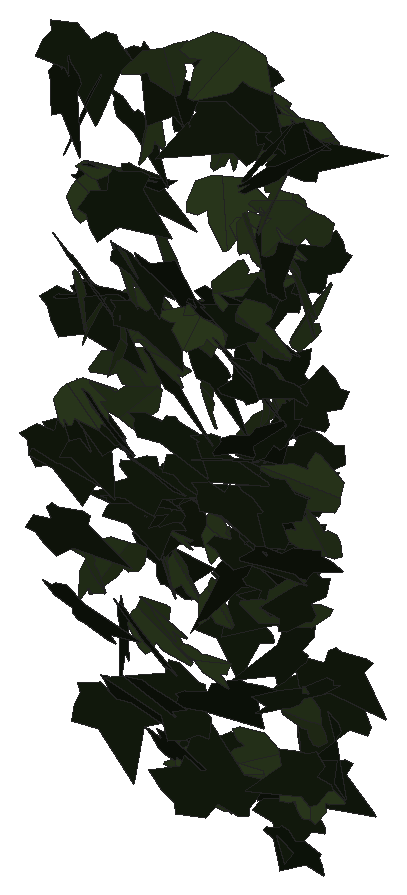
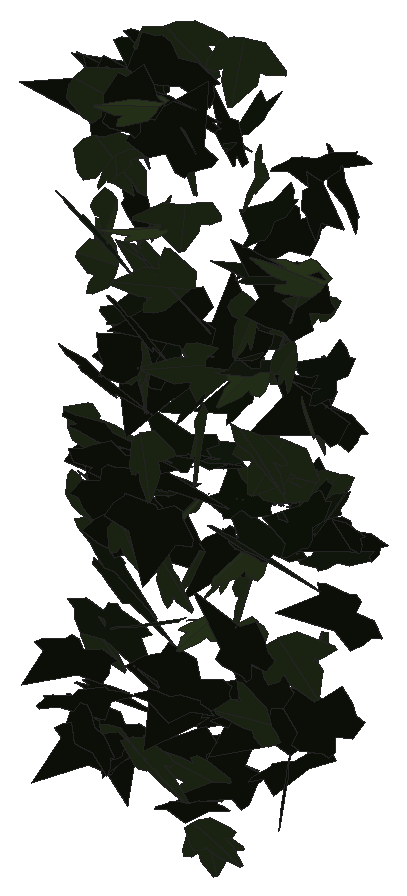
# SketchUp Ruby script. Lengths in inches.
U = 1.inch
M = Sketchup.active_model
def pt(a) = Geom::Point3d.new(a.map { |v| v * U })
def face(e, loops, mat)
  f = e.add_face(loops[0].map { |a| pt(a) })
  loops[1..].each { |l| e.add_face(l.map { |a| pt(a) }).erase! }
  f.material = f.back_material = mat if mat
  f
end
# faces: each face lists its corners as indices into pts; further lists are holes
def faces(e, pts, list, mat = nil) = list.each { |f| face(e, (f[0].is_a?(Array) ? f : [f]).map { |l| l.map { |i| pts[i] } }, mat) }
# xy, xz, yz: faces in a plane at the given z, y or x. An outline is a flat list of corners, or four numbers for a rectangle; further outlines are holes
def ring(l) = l.size == 4 ? [[l[0], l[1]], [l[2], l[1]], [l[2], l[3]], [l[0], l[3]]] : l.each_slice(2).to_a
def flat(e, list, mat, &to3) = list.each { |f| face(e, (f[0].is_a?(Array) ? f : [f]).map { |l| ring(l).map { |u, v| to3.(u, v) } }, mat) }
def xy(e, z, list, mat = nil) = flat(e, list, mat) { |x, y| [x, y, z] }
def xz(e, y, list, mat = nil) = flat(e, list, mat) { |x, z| [x, y, z] }
def yz(e, x, list, mat = nil) = flat(e, list, mat) { |y, z| [x, y, z] }
def lines(e, pts, list) = list.each { |a, b| e.add_line(pt(pts[a]), pt(pts[b])) }
# prism: a flat outline (further loops are holes) pulled along v
def prism(e, loops, v, mat = nil)
  f = face(e, loops, mat); d = Geom::Vector3d.new(v.map { |x| x * U })
  f.pushpull(f.normal.samedirection?(d) ? d.length : -d.length)
end
def box(e, o, s, mat = nil) = prism(e, [[o, [o[0] + s[0], o[1], o[2]], [o[0] + s[0], o[1] + s[1], o[2]], [o[0], o[1] + s[1], o[2]]]], [0, 0, s[2]], mat)
def at(x, y, z, deg = 0) = Geom::Transformation.translation(pt([x, y, z])) * Geom::Transformation.rotation(ORIGIN, Z_AXIS, deg.degrees)
def axes(o, x, y, z) = Geom::Transformation.new([*x, 0, *y, 0, *z, 0, *pt(o).to_a, 1])
def part(name) = M.definitions.add(name)
# library, detail: a bought-in or finely detailed component or shape, given as its bounding box
def library(name, o, s) = part(name).tap { |d| box(d.entities, o, s) }
def detail(e, o, s) = box(e.add_group.entities, o, s)
def put(e, d, t, mat = nil) = e.add_instance(d, t).tap { |i| i.material = mat if mat }
def group(e, t, mat = nil) = e.add_group.tap { |g| g.transformation = t; g.material = mat if mat }.entities
root = M.entities
M.materials.add("1026 AP 7946 SUNNY SIDE UP").color = [254, 231, 186]
M.materials.add("efeu1").color = [18, 25, 13]
M.materials.add("efeu2").color = [43, 57, 29]
c1 = part("ivyleaf_9")
p = [[1.54,2.16,1.25],[1.36,2.04,1.19],[-0.21,0.99,0.68],[-0.71,1.11,0.82],[-0.85,0.86,0.67],[-0.8,0.17,0.21],
  [-0.9,-0.01,0.1],[-0.67,-0.16,-0.02],[-0.08,-0.08,-0.05],[-0.03,-0.6,-0.4],[0.65,-0.88,-0.66],[0.83,-0.6,-0.49],
  [1.29,-0.42,-0.43],[1.8125,-0.07,-0.26],[1.21,0.44,0.15]]
faces(c1.entities,p,[[0,1,2,3,4,5,6,7,8,9,10,11,12,13,14]],"efeu1")
c2 = part("ivyleaf_10")
p = [[0,0.5,-0.03],[-0.0625,2.02,-0.43],[-0.19,2.01,-0.46],[-0.54,1.05,-0.29],[-0.52,0.625,-0.18],[-0.83,0.76,-0.28],
  [-1.16,0.64,-0.33],[-1.15,0.33,-0.24],[-0.77,-0.39,0.02],[-0.3,-0.51,0.16],[0.04,-0.48,0.23],[-0.02,2.01,-0.4375],
  [-0.06,2.01,-0.43],[0.04,-0.49,0.23],[0.67,-0.49,0.14],[1.38,0.36,-0.2],[1.375,0.51,-0.24],[0.81,0.65,-0.19],
  [0.62,0.59,-0.15],[0.6,1.09,-0.28],[0.5,1.23,-0.31]]
faces(c2.entities,p,[[0,1,2,3,4,5,6,7,8,9,10],[11,12,0,13,14,15,16,17,18,19,20]],"efeu2")
put(root,c1,axes([138.14,212.48,269.49],[0.02505,-0.04935,-0.33839],[0.43032,-0.18391,0.0411],[-0.2952,-0.27228,0.0312]),"1026 AP 7946 SUNNY SIDE UP")
put(root,c1,axes([138.08,211.28,278.25],[-0.11576,-0.04134,-0.36975],[0.55185,-0.09415,-0.06358],[-0.1333,-0.35385,0.05787]),"1026 AP 7946 SUNNY SIDE UP")
put(root,c1,axes([138.09,211.125,272.875],[-0.04513,-0.12896,-0.26193],[0.26068,0.19947,-0.1227],[0.36343,-0.15909,0.05548]),"1026 AP 7946 SUNNY SIDE UP")
put(root,c1,axes([138.07,211.5,275.36],[0.21298,-0.22745,0.17004],[0.11545,-0.14971,-0.27334],[0.42778,0.15364,-0.01089]),"1026 AP 7946 SUNNY SIDE UP")
put(root,c1,axes([138.24,211.28,273.27],[0.24543,-0.24336,-0.11417],[-0.12013,0.08073,-0.29671],[0.40202,0.1727,-0.01896]),"1026 AP 7946 SUNNY SIDE UP")
put(root,c2,axes([138.28,211.53,276.46],[0.11982,0.24934,0.17677],[0.07384,0.16359,-0.26763],[-0.4689,0.08947,0.00303]),"1026 AP 7946 SUNNY SIDE UP")
put(root,c1,axes([138.28,211.6,278.68],[-0.19065,-0.3217,-0.07903],[0.08088,0.06041,-0.35279],[0.51304,-0.12908,0.02625]),"1026 AP 7946 SUNNY SIDE UP")
put(root,c1,axes([138.22,211.24,272.4375],[-0.1155,-0.25762,0.12234],[0.21607,-0.14087,-0.22532],[0.39133,0.00174,0.16052]),"1026 AP 7946 SUNNY SIDE UP")
put(root,c2,axes([138.33,211.28,275.17],[-0.14007,0.18468,-0.20368],[0.10163,-0.18874,-0.2116],[-0.41434,-0.10872,0.01696]),"1026 AP 7946 SUNNY SIDE UP")
put(root,c1,axes([138.06,211.56,270],[0.12232,-0.15799,0.30009],[0.34901,-0.19855,-0.17264],[0.3886,0.22805,0.06059]),"1026 AP 7946 SUNNY SIDE UP")
put(root,c2,axes([138.49,211.52,274.78],[0.14246,-0.28682,0.02237],[-0.00157,-0.02479,-0.3099],[0.45249,0.09022,-0.00812]),"1026 AP 7946 SUNNY SIDE UP")
put(root,c1,axes([138.12,211.04,271.59],[0.05942,-0.00071,-0.29912],[0.34757,0.18992,0.03027],[0.29602,-0.22285,0.0245]),"1026 AP 7946 SUNNY SIDE UP")
put(root,c1,axes([138.46,211.52,278.12],[-0.21396,0.1089,-0.29729],[0.31716,-0.2081,-0.17971],[-0.36812,-0.24258,0.01796]),"1026 AP 7946 SUNNY SIDE UP")
put(root,c1,axes([138.24,211.45,274.87],[0.43413,0.10494,0.12724],[0.19824,0.01238,-0.30257],[-0.159,0.30196,-0.02983]),"1026 AP 7946 SUNNY SIDE UP")
put(root,c2,axes([138.41,211.14,273.54],[0.1753,0.2654,0.13256],[0.09978,0.11111,-0.29555],[-0.45187,0.1275,-0.01383]),"1026 AP 7946 SUNNY SIDE UP")
put(root,c1,axes([138.22,211.44,274.84],[-0.06924,-0.10451,-0.33725],[0.4358,0.18334,-0.09781],[0.31795,-0.27406,0.06062]),"1026 AP 7946 SUNNY SIDE UP")
put(root,c2,axes([138.73,211.68,271.06],[-0.25062,-0.27775,0.15338],[-0.08237,-0.14295,-0.32986],[0.48981,-0.16615,0.02301]),"1026 AP 7946 SUNNY SIDE UP")
put(root,c2,axes([138.55,211.67,276.44],[0.11538,-0.28353,-0.13782],[0.14191,0.14918,-0.27718],[0.47098,0.02452,0.11728]),"1026 AP 7946 SUNNY SIDE UP")
put(root,c1,axes([138.39,211.22,272.99],[-0.16059,-0.13449,-0.2488],[0.34992,0.11142,-0.16073],[0.25608,-0.23659,0.0636]),"1026 AP 7946 SUNNY SIDE UP")
put(root,c2,axes([138.58,211.15,271.01],[0.10369,-0.24694,-0.14257],[0.12743,0.1513,-0.2399],[0.42535,0.01487,0.10663]),"1026 AP 7946 SUNNY SIDE UP")
put(root,c1,axes([138.32,211.72,273.13],[0.25398,-0.27432,0.14838],[0.09162,-0.13442,-0.32831],[0.47965,0.17093,-0.01586]),"1026 AP 7946 SUNNY SIDE UP")
put(root,c1,axes([138.35,211.77,276.44],[0.4803,0.1176,-0.11417],[0.14524,0.06912,0.33621],[0.20936,-0.31773,0.02868]),"1026 AP 7946 SUNNY SIDE UP")
put(root,c1,axes([138.55,211.38,273.08],[-0.12662,-0.21349,0.18868],[0.1829,-0.1998,-0.18718],[0.40407,0.02354,0.14385]),"1026 AP 7946 SUNNY SIDE UP")
put(root,c2,axes([138.84,212.3,274.51],[0.44026,-0.15538,-0.11578],[-0.17091,0.03337,-0.32889],[0.24743,0.29953,-0.02117]),"1026 AP 7946 SUNNY SIDE UP")
put(root,c2,axes([138.39,211.64,276.81],[0.01233,-0.28542,0.06808],[0.43062,0.0314,0.10386],[-0.1653,0.0605,0.27563]),"1026 AP 7946 SUNNY SIDE UP")
put(root,c1,axes([138.57,211.34,273.29],[0.14869,-0.16621,0.23984],[0.16389,-0.20939,-0.19804],[0.42016,0.14049,-0.00762]),"1026 AP 7946 SUNNY SIDE UP")
put(root,c2,axes([138.79,211.6,275.57],[-0.3188,0.25604,-0.1324],[0.0996,-0.11531,-0.33647],[-0.44038,-0.21143,0.01975]),"1026 AP 7946 SUNNY SIDE UP")
put(root,c2,axes([138.9,211.67,274.05],[-0.42734,-0.1647,-0.119],[0.17193,0.04016,-0.32643],[0.26451,-0.29219,0.01993]),"1026 AP 7946 SUNNY SIDE UP")
put(root,c1,axes([138.84,211.85,277.66],[0.15388,-0.29524,0.14652],[0.07734,-0.13529,-0.3212],[0.51062,0.10946,0.00449]),"1026 AP 7946 SUNNY SIDE UP")
put(root,c2,axes([139.19,211.08,274.71],[0.06774,-0.22613,-0.27509],[-0.0059,0.26745,-0.23351],[0.54863,0.03079,0.03146]),"1026 AP 7946 SUNNY SIDE UP")
put(root,c1,axes([138.99,211.23,269.08],[-0.05416,-0.33593,-0.09017],[0.01822,0.08487,-0.34738],[0.5448,-0.03624,0.00266]),"1026 AP 7946 SUNNY SIDE UP")
put(root,c1,axes([138.77,211.71,276.77],[0.18242,-0.2912,-0.02176],[0.29401,0.09025,-0.24224],[0.35236,0.07545,0.21339]),"1026 AP 7946 SUNNY SIDE UP")
put(root,c2,axes([139.02,211.45,273.36],[-0.47276,-0.05995,0.16576],[0.24424,0.04493,0.31585],[-0.11625,0.3382,-0.0105]),"1026 AP 7946 SUNNY SIDE UP")
put(root,c2,axes([139.32,211.77,276.04],[-0.35279,0.27459,-0.0305],[0.00933,-0.03535,-0.36506],[-0.43444,-0.22374,0.01693]),"1026 AP 7946 SUNNY SIDE UP")
put(root,c1,axes([139.23,210.83,277.0625],[0.08087,-0.1191,-0.34753],[-0.12501,0.32779,-0.13006],[0.54744,0.09244,0.02164]),"1026 AP 7946 SUNNY SIDE UP")
put(root,c1,axes([139.13,211.62,275.54],[-0.01464,-0.2549,0.15671],[0.14231,-0.14878,-0.24964],[0.44575,0.03913,0.08485]),"1026 AP 7946 SUNNY SIDE UP")
put(root,c2,axes([138.98,211.91,270.02],[0.17846,-0.01013,0.32037],[0.48723,-0.02703,-0.11755],[0.04539,0.32999,0.00215]),"1026 AP 7946 SUNNY SIDE UP")
put(root,c1,axes([139.86,211.42,272.3],[-0.36261,0.21495,0.11469],[-0.25014,-0.02065,-0.30183],[-0.28573,-0.25471,0.1187]),"1026 AP 7946 SUNNY SIDE UP")
put(root,c1,axes([139.15,211.54,270.04],[0.09687,-0.18618,0.29],[0.19474,-0.25487,-0.20232],[0.49515,0.13666,0.02284]),"1026 AP 7946 SUNNY SIDE UP")
put(root,c2,axes([139.41,211.52,278],[-0.02744,0.18936,-0.3025],[0.00505,-0.29498,-0.19717],[-0.5508,-0.01214,0.01326]),"1026 AP 7946 SUNNY SIDE UP")
put(root,c1,axes([139.16,211.96,270.9],[0.01838,0.0008,0.3422],[0.30426,-0.27018,-0.00793],[0.42454,0.19359,-0.00913]),"1026 AP 7946 SUNNY SIDE UP")
put(root,c2,axes([139.71,212.22,268.23],[0.24114,0.01203,-0.19774],[-0.29567,0.06131,-0.1504],[0.06398,0.23797,0.05024]),"1026 AP 7946 SUNNY SIDE UP")
put(root,c1,axes([139.29,211.31,272.24],[0.01079,-0.2544,0.09526],[0.40952,-0.01999,-0.07551],[0.1188,0.09202,0.25164]),"1026 AP 7946 SUNNY SIDE UP")
put(root,c1,axes([139.39,211.43,275.01],[-0.01622,-0.29358,0.02374],[0.25374,-0.02632,-0.25286],[0.38759,0.00494,0.16654]),"1026 AP 7946 SUNNY SIDE UP")
put(root,c2,axes([139.7,211.35,271.6],[-0.28115,0.323,0.06868],[-0.07738,0.04675,-0.3795],[-0.5122,-0.18436,0.01963]),"1026 AP 7946 SUNNY SIDE UP")
put(root,c2,axes([139.77,212.08,268],[-0.28746,-0.15357,0.05167],[-0.01669,-0.06544,-0.24245],[0.2539,-0.17817,0.04256]),"1026 AP 7946 SUNNY SIDE UP")
put(root,c1,axes([139.51,211.22,272.15],[-0.13331,-0.26201,0.0233],[0.259,-0.0726,-0.21656],[0.32262,-0.04998,0.18348]),"1026 AP 7946 SUNNY SIDE UP")
put(root,c1,axes([139.59,211.5,278.61],[-0.08444,-0.23452,0.2963],[-0.01626,-0.29089,-0.2469],[0.58493,-0.04194,0.03591]),"1026 AP 7946 SUNNY SIDE UP")
put(root,c1,axes([139.48,210.93,269.58],[0.56042,0.01846,0.00249],[0.00553,-0.02331,-0.36701],[-0.02873,0.35566,-0.02209]),"1026 AP 7946 SUNNY SIDE UP")
put(root,c1,axes([139.58,211.69,275.32],[0.49843,-0.15639,0.01307],[0.01413,0.04862,0.36112],[-0.24643,-0.31353,0.04715]),"1026 AP 7946 SUNNY SIDE UP")
put(root,c1,axes([139.49,210.99,272.74],[0.34919,-0.12692,-0.10675],[0.15958,0.24323,-0.082],[0.20136,0.02735,0.25012]),"1026 AP 7946 SUNNY SIDE UP")
put(root,c2,axes([139.74,211.28,271.99],[0.38544,-0.11025,-0.02357],[0.14913,0.2313,-0.10293],[0.09508,0.08418,0.257]),"1026 AP 7946 SUNNY SIDE UP")
put(root,c2,axes([139.79,211.11,274.65],[0.36177,-0.14443,-0.09017],[0.16548,0.23784,-0.11906],[0.20683,0.06233,0.25297]),"1026 AP 7946 SUNNY SIDE UP")
put(root,c2,axes([139.79,211.1,270.75],[0.31924,-0.17192,-0.03917],[0.18977,0.17735,-0.16549],[0.20114,0.10553,0.2183]),"1026 AP 7946 SUNNY SIDE UP")
put(root,c1,axes([139.9,211.35,272.16],[0.04552,-0.08165,-0.33252],[-0.16559,0.30462,-0.08746],[0.49589,0.10922,0.00132]),"1026 AP 7946 SUNNY SIDE UP")
put(root,c1,axes([139.77,211.51,278.27],[-0.04484,0.11316,0.34125],[0.11634,-0.32223,0.11831],[0.53699,0.07926,0.00286]),"1026 AP 7946 SUNNY SIDE UP")
put(root,c1,axes([140.21,211.35,269.42],[-0.06087,-0.30383,-0.17047],[-0.04779,-0.16113,0.31447],[-0.5406,0.04846,-0.0086]),"1026 AP 7946 SUNNY SIDE UP")
put(root,c1,axes([139.83,211.27,272.7],[-0.17976,-0.15277,0.20946],[0.22563,-0.22352,-0.09083],[0.33149,0.06929,0.17541]),"1026 AP 7946 SUNNY SIDE UP")
put(root,c2,axes([140.18,211.71,274.01],[-0.17059,0.2054,0.31866],[-0.2975,0.24529,-0.23562],[-0.50058,-0.21578,0.03145]),"1026 AP 7946 SUNNY SIDE UP")
put(root,c1,axes([139.76,211.3,273.52],[0.05298,-0.28101,0.02989],[0.24838,-0.00684,-0.24392],[0.3686,0.045,0.16007]),"1026 AP 7946 SUNNY SIDE UP")
put(root,c2,axes([140.07,210.96,279.4],[-0.30522,-0.28796,-0.0895],[0.09253,0.06306,-0.35713],[0.46305,-0.2024,0.01237]),"1026 AP 7946 SUNNY SIDE UP")
put(root,c1,axes([139.79,211.1875,274.5],[0.35879,-0.26876,0.00833],[-0.01819,-0.0224,-0.36254],[0.42248,0.22728,-0.02268]),"1026 AP 7946 SUNNY SIDE UP")
put(root,c1,axes([139.85,211.25,268.73],[0.52243,-0.10884,-0.00382],[-0.02109,-0.03106,-0.35868],[0.1699,0.33081,-0.03277]),"1026 AP 7946 SUNNY SIDE UP")
put(root,c1,axes([140.05,212.12,268.47],[-0.16903,-0.21532,-0.06335],[0.094,0.03676,-0.24493],[0.33879,-0.11763,0.03636]),"1026 AP 7946 SUNNY SIDE UP")
put(root,c2,axes([140.125,211.58,275.07],[-0.41749,-0.06562,0.0837],[0.11697,-0.27475,0.02014],[0.11591,0.04092,0.28116]),"1026 AP 7946 SUNNY SIDE UP")
put(root,c1,axes([140.14,212.41,270.1875],[-0.24686,-0.17228,-0.11417],[0.15602,0.05681,-0.23755],[0.28084,-0.18299,0.03162]),"1026 AP 7946 SUNNY SIDE UP")
put(root,c2,axes([140.13,211.13,271.59],[0.12197,-0.25969,0.00642],[0.25745,0.04262,-0.21803],[0.31719,0.06527,0.17449]),"1026 AP 7946 SUNNY SIDE UP")
put(root,c2,axes([140.05,211.6875,274.96],[-0.01957,-0.03128,-0.35888],[0.41475,0.22781,-0.02947],[0.36075,-0.26361,0.01441]),"1026 AP 7946 SUNNY SIDE UP")
put(root,c2,axes([140.73,211.79,271.65],[-0.03537,0.04489,0.34535],[-0.46826,0.15611,-0.04124],[-0.25129,-0.29723,0.02824]),"1026 AP 7946 SUNNY SIDE UP")
put(root,c1,axes([140.15,211.68,274.55],[0.26741,-0.30567,0.00737],[-0.01576,-0.01574,-0.36005],[0.48058,0.16957,-0.01591]),"1026 AP 7946 SUNNY SIDE UP")
put(root,c1,axes([140.67,211.8,278.07],[0.39509,-0.17218,0.24561],[-0.27915,0.1628,0.31354],[-0.37022,-0.3065,0.0257]),"1026 AP 7946 SUNNY SIDE UP")
put(root,c1,axes([140.22,211.25,273.24],[0.28709,-0.15386,-0.16894],[0.19888,0.24436,-0.09017],[0.29113,-0.01521,0.22819]),"1026 AP 7946 SUNNY SIDE UP")
put(root,c2,axes([140.48,211.68,277.15],[0.37419,0.27738,-0.01152],[0.0156,-0.02529,-0.37584],[-0.43633,0.23697,-0.02332]),"1026 AP 7946 SUNNY SIDE UP")
put(root,c2,axes([140.67,211.57,278.21],[0.38108,-0.26999,-0.08722],[-0.05578,0.07958,-0.37233],[0.44068,0.24355,0.0283]),"1026 AP 7946 SUNNY SIDE UP")
put(root,c1,axes([140.72,211.97,272.61],[0.18189,0.31342,0.00645],[0.02974,-0.00221,-0.34365],[-0.49197,0.11574,-0.01839]),"1026 AP 7946 SUNNY SIDE UP")
put(root,c2,axes([140.29,211.35,268.38],[0.19625,-0.05228,-0.32941],[0.50779,-0.00345,0.13054],[-0.03503,-0.34295,0.04685]),"1026 AP 7946 SUNNY SIDE UP")
put(root,c1,axes([140.91,211,268.34],[-0.57074,-0.02342,0.09581],[0.14521,0.01481,0.3747],[-0.04145,0.37444,-0.00662]),"1026 AP 7946 SUNNY SIDE UP")
put(root,c1,axes([141.04,211.42,278.55],[-0.58901,0.00766,0.03722],[-0.05796,-0.06413,-0.38059],[-0.00214,-0.37082,0.06435]),"1026 AP 7946 SUNNY SIDE UP")
put(root,c1,axes([140.63,211.23,269.76],[0.40952,0.28423,0.05366],[0.08425,0.0192,-0.39611],[-0.44603,0.26459,-0.02556]),"1026 AP 7946 SUNNY SIDE UP")
put(root,c2,axes([140.79,212.14,273.65],[-0.0358,-0.33498,-0.04705],[0.02262,0.04287,-0.34544],[0.53072,-0.02443,0.01155]),"1026 AP 7946 SUNNY SIDE UP")
put(root,c1,axes([140.375,211.52,275.47],[0.47645,-0.01557,0.15029],[0.22519,-0.04214,-0.31115],[0.05067,0.33368,-0.0303]),"1026 AP 7946 SUNNY SIDE UP")
put(root,c2,axes([140.71,210.89,270.42],[0.35428,-0.08749,-0.10752],[0.11167,0.24741,-0.05453],[0.18201,0.01849,0.24273]),"1026 AP 7946 SUNNY SIDE UP")
put(root,c2,axes([140.92,211.32,279.55],[0.48144,0.1428,-0.18495],[-0.24482,-0.09235,-0.34821],[-0.26626,0.34313,-0.01425]),"1026 AP 7946 SUNNY SIDE UP")
put(root,c1,axes([140.87,212.16,270.92],[-0.34981,-0.19482,0.12775],[0.00187,-0.17447,-0.27871],[0.36406,-0.1863,0.12418]),"1026 AP 7946 SUNNY SIDE UP")
put(root,c1,axes([140.57,211.42,273.24],[0.01052,-0.24459,0.13147],[0.42673,-0.01896,-0.05165],[0.08347,0.12778,0.24749]),"1026 AP 7946 SUNNY SIDE UP")
put(root,c2,axes([140.8,211,271.41],[0.04564,-0.25656,-0.10083],[0.1876,0.09912,-0.23412],[0.38799,-0.01775,0.12506]),"1026 AP 7946 SUNNY SIDE UP")
put(root,c2,axes([141.14,211.77,268.75],[0.32537,-0.14152,-0.23305],[-0.33073,0.08802,-0.25532],[0.25645,0.29306,-0.03359]),"1026 AP 7946 SUNNY SIDE UP")
put(root,c2,axes([140.77,211.09,272.33],[0.11575,-0.24931,-0.11299],[0.2497,0.13048,-0.19754],[0.34685,-0.01074,0.17991]),"1026 AP 7946 SUNNY SIDE UP")
put(root,c2,axes([140.79,211.47,275.81],[-0.03506,-0.08383,0.36518],[0.16226,0.33963,0.0913],[-0.55005,0.10554,0.00366]),"1026 AP 7946 SUNNY SIDE UP")
put(root,c1,axes([140.96,212.27,275.64],[-0.38547,-0.01382,-0.21406],[0.3228,-0.0692,-0.24527],[-0.05421,-0.31377,0.06159]),"1026 AP 7946 SUNNY SIDE UP")
put(root,c2,axes([141.125,212.14,272.3],[-0.12811,-0.25003,0.05619],[-0.02049,-0.05461,-0.27119],[0.40235,-0.08239,0.00408]),"1026 AP 7946 SUNNY SIDE UP")
put(root,c1,axes([141.44,211.16,275.74],[-0.259,0.24422,0.17945],[-0.17874,0.13138,-0.30214],[-0.43514,-0.19933,0.0173]),"1026 AP 7946 SUNNY SIDE UP")
put(root,c2,axes([141.26,211.59,274.35],[0.0571,-0.0499,-0.3469],[-0.14899,0.32348,-0.05807],[0.51365,0.09938,0.02172]),"1026 AP 7946 SUNNY SIDE UP")
put(root,c1,axes([140.79,211.46,279.28],[-0.19272,-0.11132,-0.35287],[0.48336,0.15493,-0.16459],[0.29328,-0.3285,0.03938]),"1026 AP 7946 SUNNY SIDE UP")
put(root,c1,axes([141.34,212.3125,273],[-0.00875,0.0416,-0.31349],[-0.07332,-0.30118,-0.04327],[-0.47771,0.04546,0.01238]),"1026 AP 7946 SUNNY SIDE UP")
put(root,c1,axes([141.25,211.28,272.03],[-0.17215,0.17812,-0.37522],[0.24793,-0.33,-0.21642],[-0.58888,-0.19101,0.01857]),"1026 AP 7946 SUNNY SIDE UP")
put(root,c1,axes([141.24,211.66,274.47],[0.27965,0.14408,0.32587],[-0.43435,-0.15558,0.2327],[0.32982,-0.32706,0.03015]),"1026 AP 7946 SUNNY SIDE UP")
put(root,c2,axes([141.02,211.48,276.86],[0.12734,-0.29288,0.03643],[0.27639,0.017,-0.25749],[0.37293,0.08741,0.1784]),"1026 AP 7946 SUNNY SIDE UP")
put(root,c1,axes([141.72,211.28,272.73],[-0.31864,0.15198,0.29533],[-0.40693,0.1265,-0.25758],[-0.30576,-0.32673,0.03503]),"1026 AP 7946 SUNNY SIDE UP")
put(root,c1,axes([140.96,211.13,272.94],[0.04812,-0.28216,-0.00501],[0.19662,0.0165,-0.26185],[0.39775,0.02598,0.13005]),"1026 AP 7946 SUNNY SIDE UP")
put(root,c2,axes([140.9,211.75,276.74],[0.01168,-0.29031,-0.05072],[0.45243,0.01709,-0.06099],[0.09633,-0.04503,0.29261]),"1026 AP 7946 SUNNY SIDE UP")
put(root,c2,axes([140.91,211.93,278.68],[0.01241,-0.29786,0.0579],[0.46755,-0.00394,-0.0627],[0.09506,0.05829,0.30084]),"1026 AP 7946 SUNNY SIDE UP")
put(root,c1,axes([140.92,211.33,274.9],[0.35717,-0.26019,0.11398],[0.1003,-0.09305,-0.35613],[0.43406,0.2356,-0.0115]),"1026 AP 7946 SUNNY SIDE UP")
put(root,c1,axes([141.57,212.09,271.88],[-0.32439,0.25682,0.01357],[-0.02804,0.00069,-0.33908],[-0.40327,-0.20664,0.01266]),"1026 AP 7946 SUNNY SIDE UP")
put(root,c1,axes([141.78,211.91,272.91],[-0.19105,0.01738,0.31312],[-0.47675,-0.03525,-0.12303],[0.04145,-0.32533,0.02812]),"1026 AP 7946 SUNNY SIDE UP")
put(root,c2,axes([141.3,211.63,274.65],[-0.34037,0.20551,-0.17016],[0.15762,-0.13514,-0.30718],[-0.3847,-0.2372,0.0247]),"1026 AP 7946 SUNNY SIDE UP")
put(root,c1,axes([141.26,211.86,272.07],[0.26978,0.25064,0.07792],[-0.08716,-0.05186,0.31217],[0.40167,-0.17959,0.0154]),"1026 AP 7946 SUNNY SIDE UP")
put(root,c1,axes([141.22,211,272.375],[0.23326,-0.22482,-0.04524],[0.21519,0.12789,-0.20344],[0.28837,0.08642,0.1884]),"1026 AP 7946 SUNNY SIDE UP")
put(root,c1,axes([141.21,211.77,278.44],[0.10874,-0.09938,0.33672],[0.30984,-0.26152,-0.12618],[0.43985,0.20879,0.00564]),"1026 AP 7946 SUNNY SIDE UP")
put(root,c1,axes([141.58,210.9,274.15],[0.28472,0.32609,0.03348],[0.04992,0.01738,-0.38364],[-0.51258,0.18283,-0.01876]),"1026 AP 7946 SUNNY SIDE UP")
put(root,c1,axes([142.04,211.85,274.3],[-0.2252,0.17725,0.22042],[-0.27619,0.12731,-0.23011],[-0.33693,-0.22283,0.0413]),"1026 AP 7946 SUNNY SIDE UP")
put(root,c1,axes([142.08,211.84,273.4],[-0.35148,0.09576,0.19486],[-0.30587,0.01472,-0.24511],[-0.13064,-0.2921,0.04963]),"1026 AP 7946 SUNNY SIDE UP")
put(root,c2,axes([141.35,211.15,275.69],[-0.05347,0.01278,-0.36421],[0.40742,-0.24102,-0.03605],[-0.3789,-0.26097,0.01264]),"1026 AP 7946 SUNNY SIDE UP")
put(root,c1,axes([141.5,211.32,276.48],[-0.06801,0.12337,0.32423],[0.1228,-0.30433,0.13248],[0.5161,0.08867,0.0112]),"1026 AP 7946 SUNNY SIDE UP")
put(root,c1,axes([141.83,210.78,278.45],[0.06091,0.2341,0.28778],[0.06066,0.27536,-0.24279],[-0.56825,0.05449,0.00493]),"1026 AP 7946 SUNNY SIDE UP")
put(root,c1,axes([141.79,212.38,269.62],[-0.31901,-0.27814,0.01897],[0.00646,-0.0277,-0.35425],[0.43842,-0.20197,0.01902]),"1026 AP 7946 SUNNY SIDE UP")
put(root,c2,axes([141.78,211.24,277.95],[0.27918,-0.3283,0.07863],[0.0369,-0.07613,-0.38463],[0.52938,0.17844,-0.01466]),"1026 AP 7946 SUNNY SIDE UP")
put(root,c2,axes([142.07,211.69,278.49],[-0.18573,-0.12678,0.29938],[-0.27809,-0.23197,-0.17922],[0.41503,-0.21217,0.01389]),"1026 AP 7946 SUNNY SIDE UP")
put(root,c1,axes([141.73,211.27,274.91],[-0.27422,-0.1704,0.15055],[0.1571,-0.22534,-0.1482],[0.31719,-0.03571,0.20355]),"1026 AP 7946 SUNNY SIDE UP")
put(root,c1,axes([141.53,212.3125,269.2],[-0.12868,-0.02831,-0.34268],[0.52461,-0.0126,-0.08357],[-0.00867,-0.34217,0.02941]),"1026 AP 7946 SUNNY SIDE UP")
put(root,c2,axes([142.01,211.82,272.23],[-0.4325,0.02941,-0.13016],[-0.18941,0.05305,0.28282],[0.07638,0.29807,-0.03567]),"1026 AP 7946 SUNNY SIDE UP")
put(root,c2,axes([141.71,211.57,277.41],[-0.13744,-0.25271,0.14935],[0.21933,-0.17039,-0.21819],[0.40348,0.00654,0.16948]),"1026 AP 7946 SUNNY SIDE UP")
put(root,c1,axes([142.11,211.24,270.92],[-0.39841,0.23627,-0.03777],[0.00813,-0.04993,-0.35559],[-0.3762,-0.2513,0.03231]),"1026 AP 7946 SUNNY SIDE UP")
put(root,c1,axes([141.82,211.29,268.67],[0.22601,0.20269,0.0041],[0.00674,0.00042,-0.25596],[-0.31867,0.14376,-0.00251]),"1026 AP 7946 SUNNY SIDE UP")
put(root,c1,axes([142.17,211.72,276.49],[-0.16716,0.23903,0.20682],[-0.197,0.16003,-0.2655],[-0.44806,-0.15954,0.03958]),"1026 AP 7946 SUNNY SIDE UP")
put(root,c1,axes([141.64,211.12,271.74],[0.4171,0.00354,-0.02426],[0.0029,0.25953,0.06311],[0.03737,-0.05971,0.26591]),"1026 AP 7946 SUNNY SIDE UP")
put(root,c2,axes([142.07,211.39,277.42],[-0.37323,-0.18549,0.19948],[-0.18747,-0.16017,-0.3079],[0.37899,-0.2619,0.04414]),"1026 AP 7946 SUNNY SIDE UP")
put(root,c1,axes([142.18,211.23,270.23],[-0.11823,0.33367,0.01449],[-0.19236,-0.01592,-0.32898],[-0.4885,-0.07448,0.12603]),"1026 AP 7946 SUNNY SIDE UP")
put(root,c1,axes([142,210.875,274.21],[-0.29481,0.21347,-0.14265],[-0.15326,0.10026,0.29321],[0.37071,0.21121,0.00778]),"1026 AP 7946 SUNNY SIDE UP")
put(root,c2,axes([142.26,211.62,273.24],[0.03162,0.04929,0.32733],[-0.47978,-0.09659,0.0348],[0.15805,-0.30307,0.04015]),"1026 AP 7946 SUNNY SIDE UP")
put(root,c1,axes([141.7,210.82,278.1],[0.092,0.34175,-0.0865],[0.01265,0.08576,0.35763],[0.55394,-0.05872,0.0062]),"1026 AP 7946 SUNNY SIDE UP")
put(root,c1,axes([141.91,211.42,268.37],[-0.19833,-0.2114,-0.02256],[0.03999,0.00887,-0.25293],[0.33159,-0.12751,0.01701]),"1026 AP 7946 SUNNY SIDE UP")
put(root,c2,axes([141.94,211.18,271.43],[-0.4085,-0.24719,0.03114],[0.01836,0.03358,0.36925],[-0.39143,0.25955,-0.01519]),"1026 AP 7946 SUNNY SIDE UP")
put(root,c2,axes([142.05,211.38,275.69],[0.14034,-0.21301,0.31276],[-0.13444,0.29331,0.23867],[-0.56905,-0.12183,0.02075]),"1026 AP 7946 SUNNY SIDE UP")
put(root,c1,axes([141.84,212.18,270.2],[-0.04529,-0.11034,-0.28153],[0.14127,0.25757,-0.11565],[0.4404,-0.09397,0.00815]),"1026 AP 7946 SUNNY SIDE UP")
put(root,c2,axes([142.04,211.34,276.48],[-0.33721,0.30678,0.0003],[-0.01883,-0.01014,-0.38533],[-0.48201,-0.21422,0.01484]),"1026 AP 7946 SUNNY SIDE UP")
put(root,c1,axes([141.91,211.74,268.69],[0.01016,-0.05992,-0.33747],[-0.03058,0.32668,-0.06011],[0.52222,0.0203,0.00305]),"1026 AP 7946 SUNNY SIDE UP")
put(root,c2,axes([142.38,211.26,269.92],[-0.1249,0.05325,0.28528],[-0.42179,0.07344,-0.09349],[-0.13522,-0.27826,0.02812]),"1026 AP 7946 SUNNY SIDE UP")
put(root,c1,axes([141.67,211.43,278.24],[0.21099,0.05063,0.33776],[0.51187,0.04639,-0.14449],[-0.0981,0.35094,-0.0275]),"1026 AP 7946 SUNNY SIDE UP")
put(root,c1,axes([142.13,210.89,272.54],[0.32259,0.24112,-0.11199],[-0.09099,-0.0951,-0.32625],[-0.40672,0.21251,-0.01584]),"1026 AP 7946 SUNNY SIDE UP")
put(root,c1,axes([142.21,211.04,268.125],[0.23328,0.04297,-0.19956],[-0.28405,-0.07154,-0.1591],[-0.12997,0.23348,-0.01048]),"1026 AP 7946 SUNNY SIDE UP")
put(root,c1,axes([142.36,211.26,269.08],[-0.37079,0.00328,0.08972],[-0.13592,-0.04049,-0.23983],[0.01728,-0.24809,0.03884]),"1026 AP 7946 SUNNY SIDE UP")
put(root,c2,axes([142.03,211.54,268.66],[0.32618,0.13433,0.01565],[0.03125,-0.00419,-0.2542],[-0.21013,0.2079,-0.01351]),"1026 AP 7946 SUNNY SIDE UP")
put(root,c1,axes([142.49,210.96,271.91],[-0.32592,0.2253,0.12285],[-0.17946,0.0536,-0.31172],[-0.35736,-0.23239,0.0445]),"1026 AP 7946 SUNNY SIDE UP")
